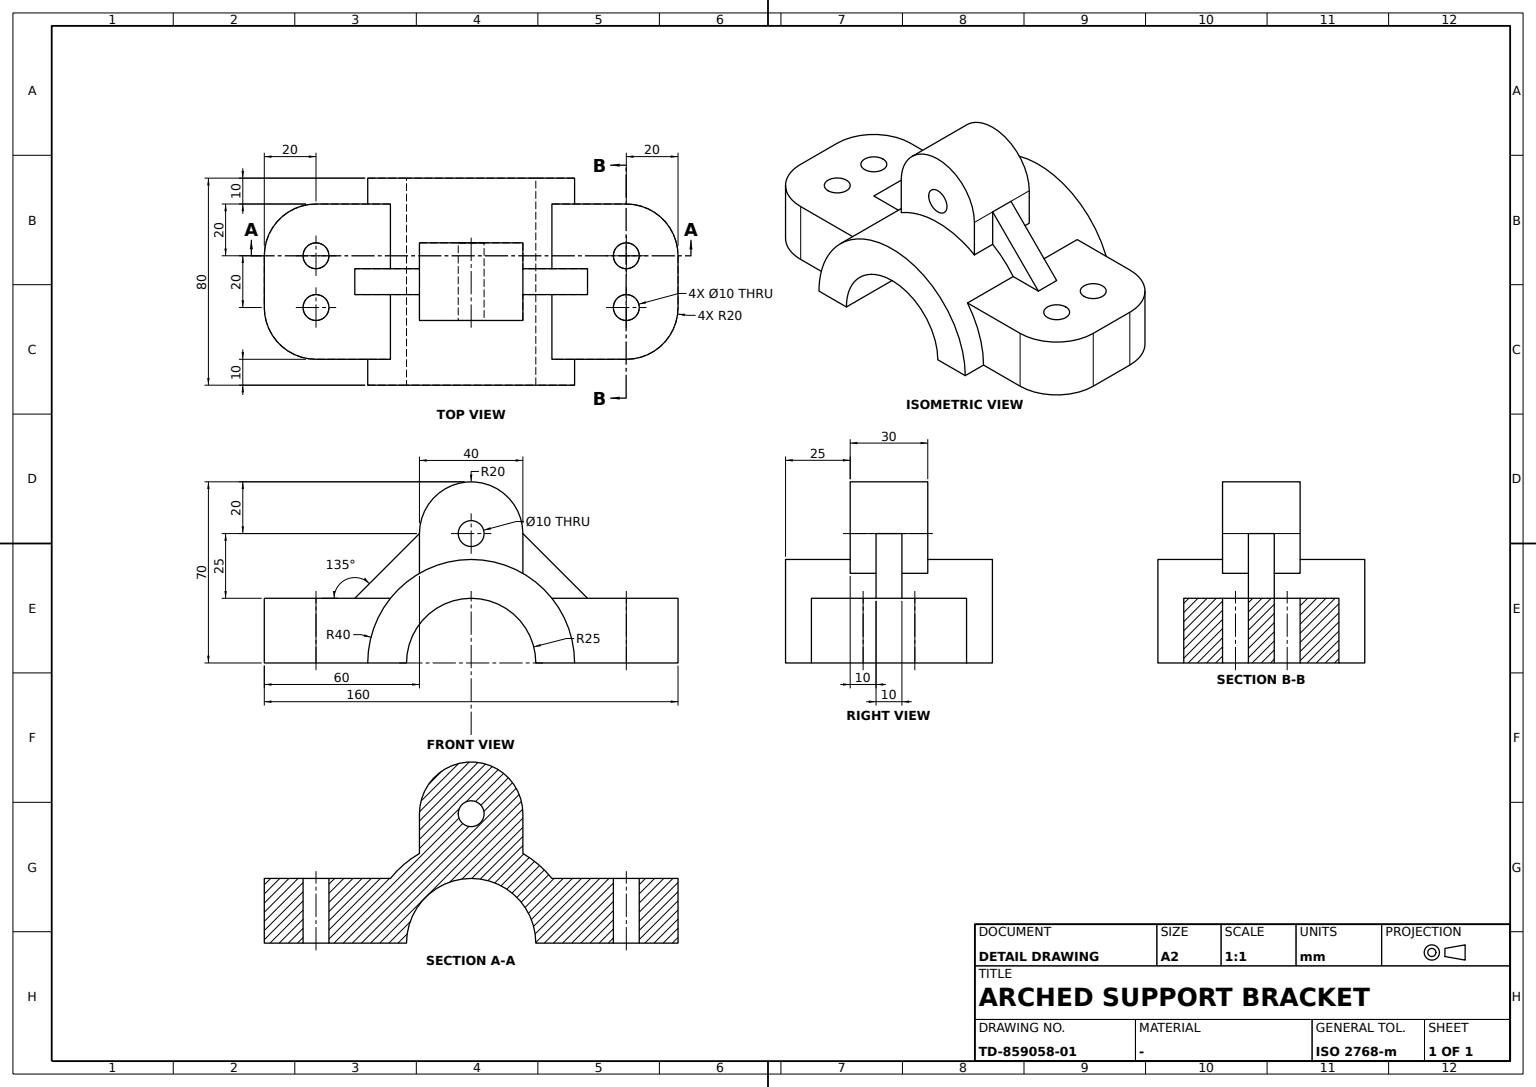
ISO-10303-21;
HEADER;
FILE_DESCRIPTION((''),'2;1');
FILE_NAME('','',(''),(''),'','','');
FILE_SCHEMA(('AUTOMOTIVE_DESIGN'));
ENDSEC;
DATA;
#1=APPLICATION_CONTEXT('');
#2=PRODUCT_CONTEXT('',#1,'mechanical');
#3=PRODUCT('','','',(#2));
#4=PRODUCT_DEFINITION_FORMATION('','',#3);
#5=PRODUCT_DEFINITION_CONTEXT('',#1,'design');
#6=PRODUCT_DEFINITION('','',#4,#5);
#7=PRODUCT_DEFINITION_SHAPE('','',#6);
#8=(LENGTH_UNIT()NAMED_UNIT(*)SI_UNIT(.MILLI.,.METRE.));
#9=(NAMED_UNIT(*)PLANE_ANGLE_UNIT()SI_UNIT($,.RADIAN.));
#10=(NAMED_UNIT(*)SI_UNIT($,.STERADIAN.)SOLID_ANGLE_UNIT());
#11=UNCERTAINTY_MEASURE_WITH_UNIT(LENGTH_MEASURE(1.E-05),#8,'distance_accuracy_value','');
#12=(GEOMETRIC_REPRESENTATION_CONTEXT(3)GLOBAL_UNCERTAINTY_ASSIGNED_CONTEXT((#11))GLOBAL_UNIT_ASSIGNED_CONTEXT((#8,#9,#10))REPRESENTATION_CONTEXT('',''));
#13=CARTESIAN_POINT('',(40.,25.,0.));
#14=VERTEX_POINT('',#13);
#15=CARTESIAN_POINT('',(40.,-25.,0.));
#16=VERTEX_POINT('',#15);
#17=CARTESIAN_POINT('',(40.,0.,0.));
#18=DIRECTION('',(1.,0.,0.));
#19=DIRECTION('',(0.,1.,0.));
#20=AXIS2_PLACEMENT_3D('',#17,#18,#19);
#21=CIRCLE('',#20,25.);
#22=EDGE_CURVE('',#14,#16,#21,.T.);
#23=ORIENTED_EDGE('',*,*,#22,.F.);
#24=CARTESIAN_POINT('',(40.,40.,0.));
#25=VERTEX_POINT('',#24);
#26=CARTESIAN_POINT('',(40.,32.5,0.));
#27=VECTOR('',#19,1000.);
#28=LINE('',#26,#27);
#29=EDGE_CURVE('',#14,#25,#28,.T.);
#30=ORIENTED_EDGE('',*,*,#29,.T.);
#31=CARTESIAN_POINT('',(40.,-40.,0.));
#32=VERTEX_POINT('',#31);
#33=CIRCLE('',#20,40.);
#34=EDGE_CURVE('',#25,#32,#33,.T.);
#35=ORIENTED_EDGE('',*,*,#34,.T.);
#36=CARTESIAN_POINT('',(40.,-32.5,0.));
#37=LINE('',#36,#27);
#38=EDGE_CURVE('',#32,#16,#37,.T.);
#39=ORIENTED_EDGE('',*,*,#38,.T.);
#40=EDGE_LOOP('',(#23,#30,#35,#39));
#41=FACE_OUTER_BOUND('',#40,.T.);
#42=PLANE('',#20);
#43=ADVANCED_FACE('',(#41),#42,.T.);
#44=CARTESIAN_POINT('',(15.,-5.,50.));
#45=VERTEX_POINT('',#44);
#46=CARTESIAN_POINT('',(-15.,-5.,50.));
#47=VERTEX_POINT('',#46);
#48=CARTESIAN_POINT('',(-13.16,-5.,50.));
#49=DIRECTION('',(-1.,0.,0.));
#50=VECTOR('',#49,1000.);
#51=LINE('',#48,#50);
#52=EDGE_CURVE('',#45,#47,#51,.T.);
#53=ORIENTED_EDGE('',*,*,#52,.F.);
#54=CARTESIAN_POINT('',(15.,5.,50.));
#55=VERTEX_POINT('',#54);
#56=CARTESIAN_POINT('',(15.,0.,50.));
#57=AXIS2_PLACEMENT_3D('',#56,#18,#19);
#58=CIRCLE('',#57,5.);
#59=EDGE_CURVE('',#45,#55,#58,.T.);
#60=ORIENTED_EDGE('',*,*,#59,.T.);
#61=CARTESIAN_POINT('',(-15.,5.,50.));
#62=VERTEX_POINT('',#61);
#63=CARTESIAN_POINT('',(-13.16,5.,50.));
#64=LINE('',#63,#50);
#65=EDGE_CURVE('',#55,#62,#64,.T.);
#66=ORIENTED_EDGE('',*,*,#65,.T.);
#67=CARTESIAN_POINT('',(-15.,0.,50.));
#68=AXIS2_PLACEMENT_3D('',#67,#18,#19);
#69=CIRCLE('',#68,5.);
#70=EDGE_CURVE('',#47,#62,#69,.T.);
#71=ORIENTED_EDGE('',*,*,#70,.F.);
#72=EDGE_LOOP('',(#53,#60,#66,#71));
#73=FACE_OUTER_BOUND('',#72,.T.);
#74=CARTESIAN_POINT('',(-13.16,0.,50.));
#75=AXIS2_PLACEMENT_3D('',#74,#49,#19);
#76=CYLINDRICAL_SURFACE('',#75,5.);
#77=ADVANCED_FACE('',(#73),#76,.F.);
#78=CARTESIAN_POINT('',(-5.,60.,0.));
#79=VERTEX_POINT('',#78);
#80=CARTESIAN_POINT('',(-15.,60.,0.));
#81=VERTEX_POINT('',#80);
#82=CARTESIAN_POINT('',(-10.,60.,0.));
#83=DIRECTION('',(0.,0.,-1.));
#84=AXIS2_PLACEMENT_3D('',#82,#83,#19);
#85=CIRCLE('',#84,5.);
#86=EDGE_CURVE('',#79,#81,#85,.T.);
#87=ORIENTED_EDGE('',*,*,#86,.T.);
#88=CARTESIAN_POINT('',(-15.,60.,25.));
#89=VERTEX_POINT('',#88);
#90=CARTESIAN_POINT('',(-15.,60.,11.84));
#91=VECTOR('',#83,1000.);
#92=LINE('',#90,#91);
#93=EDGE_CURVE('',#89,#81,#92,.T.);
#94=ORIENTED_EDGE('',*,*,#93,.F.);
#95=CARTESIAN_POINT('',(-5.,60.,25.));
#96=VERTEX_POINT('',#95);
#97=CARTESIAN_POINT('',(-10.,60.,25.));
#98=DIRECTION('',(0.,0.,1.));
#99=AXIS2_PLACEMENT_3D('',#97,#98,#18);
#100=CIRCLE('',#99,5.);
#101=EDGE_CURVE('',#89,#96,#100,.T.);
#102=ORIENTED_EDGE('',*,*,#101,.T.);
#103=CARTESIAN_POINT('',(-5.,60.,11.84));
#104=LINE('',#103,#91);
#105=EDGE_CURVE('',#96,#79,#104,.T.);
#106=ORIENTED_EDGE('',*,*,#105,.T.);
#107=EDGE_LOOP('',(#87,#94,#102,#106));
#108=FACE_OUTER_BOUND('',#107,.T.);
#109=CARTESIAN_POINT('',(-10.,60.,11.84));
#110=AXIS2_PLACEMENT_3D('',#109,#83,#18);
#111=CYLINDRICAL_SURFACE('',#110,5.);
#112=ADVANCED_FACE('',(#108),#111,.F.);
#113=CARTESIAN_POINT('',(5.,20.,50.));
#114=VERTEX_POINT('',#113);
#115=CARTESIAN_POINT('',(5.,20.,34.641016));
#116=VERTEX_POINT('',#115);
#117=CARTESIAN_POINT('',(5.,20.,42.320508));
#118=LINE('',#117,#91);
#119=EDGE_CURVE('',#114,#116,#118,.T.);
#120=ORIENTED_EDGE('',*,*,#119,.F.);
#121=CARTESIAN_POINT('',(15.,20.,50.));
#122=VERTEX_POINT('',#121);
#123=CARTESIAN_POINT('',(10.,20.,50.));
#124=VECTOR('',#18,1000.);
#125=LINE('',#123,#124);
#126=EDGE_CURVE('',#114,#122,#125,.T.);
#127=ORIENTED_EDGE('',*,*,#126,.T.);
#128=CARTESIAN_POINT('',(15.,20.,34.641016));
#129=VERTEX_POINT('',#128);
#130=CARTESIAN_POINT('',(15.,20.,42.320508));
#131=VECTOR('',#98,1000.);
#132=LINE('',#130,#131);
#133=EDGE_CURVE('',#129,#122,#132,.T.);
#134=ORIENTED_EDGE('',*,*,#133,.F.);
#135=CARTESIAN_POINT('',(0.,20.,34.641016));
#136=LINE('',#135,#124);
#137=EDGE_CURVE('',#116,#129,#136,.T.);
#138=ORIENTED_EDGE('',*,*,#137,.F.);
#139=EDGE_LOOP('',(#120,#127,#134,#138));
#140=FACE_OUTER_BOUND('',#139,.T.);
#141=CARTESIAN_POINT('',(0.,20.,50.));
#142=DIRECTION('',(0.,-1.,0.));
#143=AXIS2_PLACEMENT_3D('',#141,#142,#83);
#144=PLANE('',#143);
#145=ADVANCED_FACE('',(#140),#144,.F.);
#146=CARTESIAN_POINT('',(-30.,60.,0.));
#147=VERTEX_POINT('',#146);
#148=CARTESIAN_POINT('',(-30.,60.,25.));
#149=VERTEX_POINT('',#148);
#150=CARTESIAN_POINT('',(-30.,60.,12.5));
#151=LINE('',#150,#131);
#152=EDGE_CURVE('',#147,#149,#151,.T.);
#153=ORIENTED_EDGE('',*,*,#152,.T.);
#154=CARTESIAN_POINT('',(-10.,80.,25.));
#155=VERTEX_POINT('',#154);
#156=AXIS2_PLACEMENT_3D('',#97,#83,#142);
#157=CIRCLE('',#156,20.);
#158=EDGE_CURVE('',#149,#155,#157,.T.);
#159=ORIENTED_EDGE('',*,*,#158,.T.);
#160=CARTESIAN_POINT('',(-10.,80.,0.));
#161=VERTEX_POINT('',#160);
#162=CARTESIAN_POINT('',(-10.,80.,12.5));
#163=LINE('',#162,#131);
#164=EDGE_CURVE('',#161,#155,#163,.T.);
#165=ORIENTED_EDGE('',*,*,#164,.F.);
#166=AXIS2_PLACEMENT_3D('',#82,#98,#19);
#167=CIRCLE('',#166,20.);
#168=EDGE_CURVE('',#161,#147,#167,.T.);
#169=ORIENTED_EDGE('',*,*,#168,.T.);
#170=EDGE_LOOP('',(#153,#159,#165,#169));
#171=FACE_OUTER_BOUND('',#170,.T.);
#172=CARTESIAN_POINT('',(-10.,60.,12.5));
#173=AXIS2_PLACEMENT_3D('',#172,#83,#49);
#174=CYLINDRICAL_SURFACE('',#173,20.);
#175=ADVANCED_FACE('',(#171),#174,.T.);
#176=ORIENTED_EDGE('',*,*,#105,.F.);
#177=EDGE_CURVE('',#96,#89,#100,.T.);
#178=ORIENTED_EDGE('',*,*,#177,.T.);
#179=ORIENTED_EDGE('',*,*,#93,.T.);
#180=EDGE_CURVE('',#81,#79,#85,.T.);
#181=ORIENTED_EDGE('',*,*,#180,.T.);
#182=EDGE_LOOP('',(#176,#178,#179,#181));
#183=FACE_OUTER_BOUND('',#182,.T.);
#184=ADVANCED_FACE('',(#183),#111,.F.);
#185=ORIENTED_EDGE('',*,*,#52,.T.);
#186=EDGE_CURVE('',#62,#47,#69,.T.);
#187=ORIENTED_EDGE('',*,*,#186,.F.);
#188=ORIENTED_EDGE('',*,*,#65,.F.);
#189=EDGE_CURVE('',#55,#45,#58,.T.);
#190=ORIENTED_EDGE('',*,*,#189,.T.);
#191=EDGE_LOOP('',(#185,#187,#188,#190));
#192=FACE_OUTER_BOUND('',#191,.T.);
#193=ADVANCED_FACE('',(#192),#76,.F.);
#194=ORIENTED_EDGE('',*,*,#189,.F.);
#195=ORIENTED_EDGE('',*,*,#59,.F.);
#196=EDGE_LOOP('',(#194,#195));
#197=FACE_BOUND('',#196,.T.);
#198=CARTESIAN_POINT('',(15.,-20.,50.));
#199=VERTEX_POINT('',#198);
#200=CARTESIAN_POINT('',(15.,-20.,34.641016));
#201=VERTEX_POINT('',#200);
#202=CARTESIAN_POINT('',(15.,-20.,42.320508));
#203=LINE('',#202,#91);
#204=EDGE_CURVE('',#199,#201,#203,.T.);
#205=ORIENTED_EDGE('',*,*,#204,.T.);
#206=CARTESIAN_POINT('',(15.,0.,0.));
#207=AXIS2_PLACEMENT_3D('',#206,#49,#19);
#208=CIRCLE('',#207,40.);
#209=EDGE_CURVE('',#201,#129,#208,.T.);
#210=ORIENTED_EDGE('',*,*,#209,.T.);
#211=ORIENTED_EDGE('',*,*,#133,.T.);
#212=CIRCLE('',#57,20.);
#213=EDGE_CURVE('',#122,#199,#212,.T.);
#214=ORIENTED_EDGE('',*,*,#213,.T.);
#215=EDGE_LOOP('',(#205,#210,#211,#214));
#216=FACE_OUTER_BOUND('',#215,.T.);
#217=AXIS2_PLACEMENT_3D('',#206,#18,#19);
#218=PLANE('',#217);
#219=ADVANCED_FACE('',(#197,#216),#218,.T.);
#220=CARTESIAN_POINT('',(-15.,20.,50.));
#221=VERTEX_POINT('',#220);
#222=CARTESIAN_POINT('',(-15.,-20.,50.));
#223=VERTEX_POINT('',#222);
#224=CIRCLE('',#68,20.);
#225=EDGE_CURVE('',#221,#223,#224,.T.);
#226=ORIENTED_EDGE('',*,*,#225,.F.);
#227=CARTESIAN_POINT('',(-15.,20.,34.641016));
#228=VERTEX_POINT('',#227);
#229=CARTESIAN_POINT('',(-15.,20.,42.320508));
#230=LINE('',#229,#131);
#231=EDGE_CURVE('',#228,#221,#230,.T.);
#232=ORIENTED_EDGE('',*,*,#231,.F.);
#233=CARTESIAN_POINT('',(-15.,-20.,34.641016));
#234=VERTEX_POINT('',#233);
#235=CARTESIAN_POINT('',(-15.,0.,0.));
#236=AXIS2_PLACEMENT_3D('',#235,#49,#19);
#237=CIRCLE('',#236,40.);
#238=EDGE_CURVE('',#234,#228,#237,.T.);
#239=ORIENTED_EDGE('',*,*,#238,.F.);
#240=CARTESIAN_POINT('',(-15.,-20.,42.320508));
#241=LINE('',#240,#91);
#242=EDGE_CURVE('',#223,#234,#241,.T.);
#243=ORIENTED_EDGE('',*,*,#242,.F.);
#244=EDGE_LOOP('',(#226,#232,#239,#243));
#245=FACE_OUTER_BOUND('',#244,.T.);
#246=ORIENTED_EDGE('',*,*,#186,.T.);
#247=ORIENTED_EDGE('',*,*,#70,.T.);
#248=EDGE_LOOP('',(#246,#247));
#249=FACE_BOUND('',#248,.T.);
#250=AXIS2_PLACEMENT_3D('',#235,#18,#19);
#251=PLANE('',#250);
#252=ADVANCED_FACE('',(#245,#249),#251,.F.);
#253=CARTESIAN_POINT('',(-10.,-80.,25.));
#254=VERTEX_POINT('',#253);
#255=CARTESIAN_POINT('',(-10.,-80.,0.));
#256=VERTEX_POINT('',#255);
#257=CARTESIAN_POINT('',(-10.,-80.,12.5));
#258=LINE('',#257,#91);
#259=EDGE_CURVE('',#254,#256,#258,.T.);
#260=ORIENTED_EDGE('',*,*,#259,.T.);
#261=CARTESIAN_POINT('',(10.,-80.,0.));
#262=VERTEX_POINT('',#261);
#263=CARTESIAN_POINT('',(0.,-80.,0.));
#264=LINE('',#263,#124);
#265=EDGE_CURVE('',#256,#262,#264,.T.);
#266=ORIENTED_EDGE('',*,*,#265,.T.);
#267=CARTESIAN_POINT('',(10.,-80.,25.));
#268=VERTEX_POINT('',#267);
#269=CARTESIAN_POINT('',(10.,-80.,12.5));
#270=LINE('',#269,#91);
#271=EDGE_CURVE('',#268,#262,#270,.T.);
#272=ORIENTED_EDGE('',*,*,#271,.F.);
#273=CARTESIAN_POINT('',(0.,-80.,25.));
#274=LINE('',#273,#124);
#275=EDGE_CURVE('',#254,#268,#274,.T.);
#276=ORIENTED_EDGE('',*,*,#275,.F.);
#277=EDGE_LOOP('',(#260,#266,#272,#276));
#278=FACE_OUTER_BOUND('',#277,.T.);
#279=AXIS2_PLACEMENT_3D('',#263,#19,#98);
#280=PLANE('',#279);
#281=ADVANCED_FACE('',(#278),#280,.F.);
#282=CARTESIAN_POINT('',(-5.,-20.,50.));
#283=VERTEX_POINT('',#282);
#284=CARTESIAN_POINT('',(5.,-20.,50.));
#285=VERTEX_POINT('',#284);
#286=CARTESIAN_POINT('',(0.,-20.,50.));
#287=LINE('',#286,#124);
#288=EDGE_CURVE('',#283,#285,#287,.T.);
#289=ORIENTED_EDGE('',*,*,#288,.F.);
#290=CARTESIAN_POINT('',(-5.,-45.,25.));
#291=VERTEX_POINT('',#290);
#292=CARTESIAN_POINT('',(-5.,-32.5,37.5));
#293=DIRECTION('',(0.,-0.707106781,-0.707106781));
#294=VECTOR('',#293,1000.);
#295=LINE('',#292,#294);
#296=EDGE_CURVE('',#283,#291,#295,.T.);
#297=ORIENTED_EDGE('',*,*,#296,.T.);
#298=CARTESIAN_POINT('',(5.,-45.,25.));
#299=VERTEX_POINT('',#298);
#300=CARTESIAN_POINT('',(0.,-45.,25.));
#301=LINE('',#300,#124);
#302=EDGE_CURVE('',#291,#299,#301,.T.);
#303=ORIENTED_EDGE('',*,*,#302,.T.);
#304=CARTESIAN_POINT('',(5.,-32.5,37.5));
#305=LINE('',#304,#294);
#306=EDGE_CURVE('',#285,#299,#305,.T.);
#307=ORIENTED_EDGE('',*,*,#306,.F.);
#308=EDGE_LOOP('',(#289,#297,#303,#307));
#309=FACE_OUTER_BOUND('',#308,.T.);
#310=DIRECTION('',(0.,0.707106781,-0.707106781));
#311=DIRECTION('',(0.,0.707106781,0.707106781));
#312=AXIS2_PLACEMENT_3D('',#286,#310,#311);
#313=PLANE('',#312);
#314=ADVANCED_FACE('',(#309),#313,.F.);
#315=CARTESIAN_POINT('',(-40.,25.,0.));
#316=VERTEX_POINT('',#315);
#317=CARTESIAN_POINT('',(-40.,40.,0.));
#318=VERTEX_POINT('',#317);
#319=CARTESIAN_POINT('',(-40.,32.5,0.));
#320=LINE('',#319,#27);
#321=EDGE_CURVE('',#316,#318,#320,.T.);
#322=ORIENTED_EDGE('',*,*,#321,.F.);
#323=CARTESIAN_POINT('',(-40.,-25.,0.));
#324=VERTEX_POINT('',#323);
#325=CARTESIAN_POINT('',(-40.,0.,0.));
#326=AXIS2_PLACEMENT_3D('',#325,#18,#19);
#327=CIRCLE('',#326,25.);
#328=EDGE_CURVE('',#316,#324,#327,.T.);
#329=ORIENTED_EDGE('',*,*,#328,.T.);
#330=CARTESIAN_POINT('',(-40.,-40.,0.));
#331=VERTEX_POINT('',#330);
#332=CARTESIAN_POINT('',(-40.,-32.5,0.));
#333=LINE('',#332,#27);
#334=EDGE_CURVE('',#331,#324,#333,.T.);
#335=ORIENTED_EDGE('',*,*,#334,.F.);
#336=CIRCLE('',#326,40.);
#337=EDGE_CURVE('',#318,#331,#336,.T.);
#338=ORIENTED_EDGE('',*,*,#337,.F.);
#339=EDGE_LOOP('',(#322,#329,#335,#338));
#340=FACE_OUTER_BOUND('',#339,.T.);
#341=PLANE('',#326);
#342=ADVANCED_FACE('',(#340),#341,.F.);
#343=CARTESIAN_POINT('',(-30.,-60.,25.));
#344=VERTEX_POINT('',#343);
#345=CARTESIAN_POINT('',(-30.,-60.,0.));
#346=VERTEX_POINT('',#345);
#347=CARTESIAN_POINT('',(-30.,-60.,12.5));
#348=LINE('',#347,#91);
#349=EDGE_CURVE('',#344,#346,#348,.T.);
#350=ORIENTED_EDGE('',*,*,#349,.F.);
#351=CARTESIAN_POINT('',(-30.,-31.22499,25.));
#352=VERTEX_POINT('',#351);
#353=CARTESIAN_POINT('',(-30.,-45.612495,25.));
#354=VECTOR('',#142,1000.);
#355=LINE('',#353,#354);
#356=EDGE_CURVE('',#352,#344,#355,.T.);
#357=ORIENTED_EDGE('',*,*,#356,.F.);
#358=CARTESIAN_POINT('',(-30.,-40.,0.));
#359=VERTEX_POINT('',#358);
#360=CARTESIAN_POINT('',(-30.,0.,0.));
#361=AXIS2_PLACEMENT_3D('',#360,#18,#19);
#362=CIRCLE('',#361,40.);
#363=EDGE_CURVE('',#352,#359,#362,.T.);
#364=ORIENTED_EDGE('',*,*,#363,.T.);
#365=CARTESIAN_POINT('',(-30.,-50.,0.));
#366=LINE('',#365,#27);
#367=EDGE_CURVE('',#346,#359,#366,.T.);
#368=ORIENTED_EDGE('',*,*,#367,.F.);
#369=EDGE_LOOP('',(#350,#357,#364,#368));
#370=FACE_OUTER_BOUND('',#369,.T.);
#371=PLANE('',#361);
#372=ADVANCED_FACE('',(#370),#371,.F.);
#373=CARTESIAN_POINT('',(5.,60.,25.));
#374=VERTEX_POINT('',#373);
#375=CARTESIAN_POINT('',(15.,60.,25.));
#376=VERTEX_POINT('',#375);
#377=CARTESIAN_POINT('',(10.,60.,25.));
#378=AXIS2_PLACEMENT_3D('',#377,#98,#18);
#379=CIRCLE('',#378,5.);
#380=EDGE_CURVE('',#374,#376,#379,.T.);
#381=ORIENTED_EDGE('',*,*,#380,.T.);
#382=CARTESIAN_POINT('',(15.,60.,0.));
#383=VERTEX_POINT('',#382);
#384=CARTESIAN_POINT('',(15.,60.,11.84));
#385=LINE('',#384,#91);
#386=EDGE_CURVE('',#376,#383,#385,.T.);
#387=ORIENTED_EDGE('',*,*,#386,.T.);
#388=CARTESIAN_POINT('',(5.,60.,0.));
#389=VERTEX_POINT('',#388);
#390=CARTESIAN_POINT('',(10.,60.,0.));
#391=AXIS2_PLACEMENT_3D('',#390,#83,#19);
#392=CIRCLE('',#391,5.);
#393=EDGE_CURVE('',#383,#389,#392,.T.);
#394=ORIENTED_EDGE('',*,*,#393,.T.);
#395=CARTESIAN_POINT('',(5.,60.,11.84));
#396=LINE('',#395,#91);
#397=EDGE_CURVE('',#374,#389,#396,.T.);
#398=ORIENTED_EDGE('',*,*,#397,.F.);
#399=EDGE_LOOP('',(#381,#387,#394,#398));
#400=FACE_OUTER_BOUND('',#399,.T.);
#401=CARTESIAN_POINT('',(10.,60.,11.84));
#402=AXIS2_PLACEMENT_3D('',#401,#83,#18);
#403=CYLINDRICAL_SURFACE('',#402,5.);
#404=ADVANCED_FACE('',(#400),#403,.F.);
#405=CARTESIAN_POINT('',(-5.,45.,25.));
#406=VERTEX_POINT('',#405);
#407=CARTESIAN_POINT('',(-5.,31.22499,25.));
#408=VERTEX_POINT('',#407);
#409=CARTESIAN_POINT('',(-5.,38.112495,25.));
#410=LINE('',#409,#354);
#411=EDGE_CURVE('',#406,#408,#410,.T.);
#412=ORIENTED_EDGE('',*,*,#411,.T.);
#413=CARTESIAN_POINT('',(-5.,20.,34.641016));
#414=VERTEX_POINT('',#413);
#415=CARTESIAN_POINT('',(-5.,0.,0.));
#416=AXIS2_PLACEMENT_3D('',#415,#18,#19);
#417=CIRCLE('',#416,40.);
#418=EDGE_CURVE('',#408,#414,#417,.T.);
#419=ORIENTED_EDGE('',*,*,#418,.T.);
#420=CARTESIAN_POINT('',(-5.,20.,50.));
#421=VERTEX_POINT('',#420);
#422=CARTESIAN_POINT('',(-5.,20.,42.320508));
#423=LINE('',#422,#91);
#424=EDGE_CURVE('',#421,#414,#423,.T.);
#425=ORIENTED_EDGE('',*,*,#424,.F.);
#426=CARTESIAN_POINT('',(-5.,32.5,37.5));
#427=VECTOR('',#310,1000.);
#428=LINE('',#426,#427);
#429=EDGE_CURVE('',#421,#406,#428,.T.);
#430=ORIENTED_EDGE('',*,*,#429,.T.);
#431=EDGE_LOOP('',(#412,#419,#425,#430));
#432=FACE_OUTER_BOUND('',#431,.T.);
#433=PLANE('',#416);
#434=ADVANCED_FACE('',(#432),#433,.F.);
#435=CARTESIAN_POINT('',(5.,-20.,34.641016));
#436=VERTEX_POINT('',#435);
#437=CARTESIAN_POINT('',(5.,-31.22499,25.));
#438=VERTEX_POINT('',#437);
#439=CARTESIAN_POINT('',(5.,0.,0.));
#440=AXIS2_PLACEMENT_3D('',#439,#18,#19);
#441=CIRCLE('',#440,40.);
#442=EDGE_CURVE('',#436,#438,#441,.T.);
#443=ORIENTED_EDGE('',*,*,#442,.F.);
#444=CARTESIAN_POINT('',(5.,-20.,42.320508));
#445=LINE('',#444,#91);
#446=EDGE_CURVE('',#285,#436,#445,.T.);
#447=ORIENTED_EDGE('',*,*,#446,.F.);
#448=ORIENTED_EDGE('',*,*,#306,.T.);
#449=CARTESIAN_POINT('',(5.,-38.112495,25.));
#450=LINE('',#449,#354);
#451=EDGE_CURVE('',#438,#299,#450,.T.);
#452=ORIENTED_EDGE('',*,*,#451,.F.);
#453=EDGE_LOOP('',(#443,#447,#448,#452));
#454=FACE_OUTER_BOUND('',#453,.T.);
#455=PLANE('',#440);
#456=ADVANCED_FACE('',(#454),#455,.T.);
#457=ORIENTED_EDGE('',*,*,#386,.F.);
#458=EDGE_CURVE('',#376,#374,#379,.T.);
#459=ORIENTED_EDGE('',*,*,#458,.T.);
#460=ORIENTED_EDGE('',*,*,#397,.T.);
#461=EDGE_CURVE('',#389,#383,#392,.T.);
#462=ORIENTED_EDGE('',*,*,#461,.T.);
#463=EDGE_LOOP('',(#457,#459,#460,#462));
#464=FACE_OUTER_BOUND('',#463,.T.);
#465=ADVANCED_FACE('',(#464),#403,.F.);
#466=CARTESIAN_POINT('',(5.,45.,25.));
#467=VERTEX_POINT('',#466);
#468=CARTESIAN_POINT('',(5.,32.5,37.5));
#469=LINE('',#468,#427);
#470=EDGE_CURVE('',#114,#467,#469,.T.);
#471=ORIENTED_EDGE('',*,*,#470,.F.);
#472=ORIENTED_EDGE('',*,*,#119,.T.);
#473=CARTESIAN_POINT('',(5.,31.22499,25.));
#474=VERTEX_POINT('',#473);
#475=EDGE_CURVE('',#474,#116,#441,.T.);
#476=ORIENTED_EDGE('',*,*,#475,.F.);
#477=CARTESIAN_POINT('',(5.,38.112495,25.));
#478=LINE('',#477,#354);
#479=EDGE_CURVE('',#467,#474,#478,.T.);
#480=ORIENTED_EDGE('',*,*,#479,.F.);
#481=EDGE_LOOP('',(#471,#472,#476,#480));
#482=FACE_OUTER_BOUND('',#481,.T.);
#483=ADVANCED_FACE('',(#482),#455,.T.);
#484=CARTESIAN_POINT('',(0.,-25.,0.));
#485=LINE('',#484,#50);
#486=EDGE_CURVE('',#16,#324,#485,.T.);
#487=ORIENTED_EDGE('',*,*,#486,.T.);
#488=ORIENTED_EDGE('',*,*,#328,.F.);
#489=CARTESIAN_POINT('',(-0.66,25.,0.));
#490=LINE('',#489,#50);
#491=EDGE_CURVE('',#14,#316,#490,.T.);
#492=ORIENTED_EDGE('',*,*,#491,.F.);
#493=ORIENTED_EDGE('',*,*,#22,.T.);
#494=EDGE_LOOP('',(#487,#488,#492,#493));
#495=FACE_OUTER_BOUND('',#494,.T.);
#496=CARTESIAN_POINT('',(-0.66,0.,0.));
#497=AXIS2_PLACEMENT_3D('',#496,#49,#19);
#498=CYLINDRICAL_SURFACE('',#497,25.);
#499=ADVANCED_FACE('',(#495),#498,.F.);
#500=CARTESIAN_POINT('',(30.,-60.,25.));
#501=VERTEX_POINT('',#500);
#502=CARTESIAN_POINT('',(30.,-60.,0.));
#503=VERTEX_POINT('',#502);
#504=CARTESIAN_POINT('',(30.,-60.,12.5));
#505=LINE('',#504,#91);
#506=EDGE_CURVE('',#501,#503,#505,.T.);
#507=ORIENTED_EDGE('',*,*,#506,.F.);
#508=CARTESIAN_POINT('',(10.,-60.,25.));
#509=AXIS2_PLACEMENT_3D('',#508,#83,#142);
#510=CIRCLE('',#509,20.);
#511=EDGE_CURVE('',#501,#268,#510,.T.);
#512=ORIENTED_EDGE('',*,*,#511,.T.);
#513=ORIENTED_EDGE('',*,*,#271,.T.);
#514=CARTESIAN_POINT('',(10.,-60.,0.));
#515=AXIS2_PLACEMENT_3D('',#514,#98,#19);
#516=CIRCLE('',#515,20.);
#517=EDGE_CURVE('',#262,#503,#516,.T.);
#518=ORIENTED_EDGE('',*,*,#517,.T.);
#519=EDGE_LOOP('',(#507,#512,#513,#518));
#520=FACE_OUTER_BOUND('',#519,.T.);
#521=CARTESIAN_POINT('',(10.,-60.,12.5));
#522=AXIS2_PLACEMENT_3D('',#521,#83,#142);
#523=CYLINDRICAL_SURFACE('',#522,20.);
#524=ADVANCED_FACE('',(#520),#523,.T.);
#525=CARTESIAN_POINT('',(30.,31.22499,25.));
#526=VERTEX_POINT('',#525);
#527=CARTESIAN_POINT('',(17.5,31.22499,25.));
#528=LINE('',#527,#124);
#529=EDGE_CURVE('',#474,#526,#528,.T.);
#530=ORIENTED_EDGE('',*,*,#529,.T.);
#531=CARTESIAN_POINT('',(30.,60.,25.));
#532=VERTEX_POINT('',#531);
#533=CARTESIAN_POINT('',(30.,45.612495,25.));
#534=LINE('',#533,#354);
#535=EDGE_CURVE('',#532,#526,#534,.T.);
#536=ORIENTED_EDGE('',*,*,#535,.F.);
#537=CARTESIAN_POINT('',(10.,80.,25.));
#538=VERTEX_POINT('',#537);
#539=AXIS2_PLACEMENT_3D('',#377,#83,#142);
#540=CIRCLE('',#539,20.);
#541=EDGE_CURVE('',#538,#532,#540,.T.);
#542=ORIENTED_EDGE('',*,*,#541,.F.);
#543=CARTESIAN_POINT('',(0.,80.,25.));
#544=LINE('',#543,#124);
#545=EDGE_CURVE('',#155,#538,#544,.T.);
#546=ORIENTED_EDGE('',*,*,#545,.F.);
#547=ORIENTED_EDGE('',*,*,#158,.F.);
#548=CARTESIAN_POINT('',(-30.,31.22499,25.));
#549=VERTEX_POINT('',#548);
#550=CARTESIAN_POINT('',(-30.,45.612495,25.));
#551=LINE('',#550,#354);
#552=EDGE_CURVE('',#149,#549,#551,.T.);
#553=ORIENTED_EDGE('',*,*,#552,.T.);
#554=CARTESIAN_POINT('',(-17.5,31.22499,25.));
#555=LINE('',#554,#124);
#556=EDGE_CURVE('',#549,#408,#555,.T.);
#557=ORIENTED_EDGE('',*,*,#556,.T.);
#558=ORIENTED_EDGE('',*,*,#411,.F.);
#559=CARTESIAN_POINT('',(0.,45.,25.));
#560=LINE('',#559,#124);
#561=EDGE_CURVE('',#406,#467,#560,.T.);
#562=ORIENTED_EDGE('',*,*,#561,.T.);
#563=ORIENTED_EDGE('',*,*,#479,.T.);
#564=EDGE_LOOP('',(#530,#536,#542,#546,#547,#553,#557,#558,#562,#563));
#565=FACE_OUTER_BOUND('',#564,.T.);
#566=ORIENTED_EDGE('',*,*,#380,.F.);
#567=ORIENTED_EDGE('',*,*,#458,.F.);
#568=EDGE_LOOP('',(#566,#567));
#569=FACE_BOUND('',#568,.T.);
#570=ORIENTED_EDGE('',*,*,#101,.F.);
#571=ORIENTED_EDGE('',*,*,#177,.F.);
#572=EDGE_LOOP('',(#570,#571));
#573=FACE_BOUND('',#572,.T.);
#574=AXIS2_PLACEMENT_3D('',#543,#98,#142);
#575=PLANE('',#574);
#576=ADVANCED_FACE('',(#565,#569,#573),#575,.T.);
#577=ORIENTED_EDGE('',*,*,#296,.F.);
#578=CARTESIAN_POINT('',(-5.,-20.,34.641016));
#579=VERTEX_POINT('',#578);
#580=CARTESIAN_POINT('',(-5.,-20.,42.320508));
#581=LINE('',#580,#91);
#582=EDGE_CURVE('',#283,#579,#581,.T.);
#583=ORIENTED_EDGE('',*,*,#582,.T.);
#584=CARTESIAN_POINT('',(-5.,-31.22499,25.));
#585=VERTEX_POINT('',#584);
#586=EDGE_CURVE('',#579,#585,#417,.T.);
#587=ORIENTED_EDGE('',*,*,#586,.T.);
#588=CARTESIAN_POINT('',(-5.,-38.112495,25.));
#589=LINE('',#588,#354);
#590=EDGE_CURVE('',#585,#291,#589,.T.);
#591=ORIENTED_EDGE('',*,*,#590,.T.);
#592=EDGE_LOOP('',(#577,#583,#587,#591));
#593=FACE_OUTER_BOUND('',#592,.T.);
#594=ADVANCED_FACE('',(#593),#433,.F.);
#595=ORIENTED_EDGE('',*,*,#561,.F.);
#596=ORIENTED_EDGE('',*,*,#429,.F.);
#597=LINE('',#141,#124);
#598=EDGE_CURVE('',#421,#114,#597,.T.);
#599=ORIENTED_EDGE('',*,*,#598,.T.);
#600=ORIENTED_EDGE('',*,*,#470,.T.);
#601=EDGE_LOOP('',(#595,#596,#599,#600));
#602=FACE_OUTER_BOUND('',#601,.T.);
#603=DIRECTION('',(0.,-0.707106781,0.707106781));
#604=AXIS2_PLACEMENT_3D('',#141,#311,#603);
#605=PLANE('',#604);
#606=ADVANCED_FACE('',(#602),#605,.T.);
#607=CARTESIAN_POINT('',(10.,80.,0.));
#608=VERTEX_POINT('',#607);
#609=CARTESIAN_POINT('',(0.,80.,0.));
#610=LINE('',#609,#124);
#611=EDGE_CURVE('',#161,#608,#610,.T.);
#612=ORIENTED_EDGE('',*,*,#611,.F.);
#613=ORIENTED_EDGE('',*,*,#164,.T.);
#614=ORIENTED_EDGE('',*,*,#545,.T.);
#615=CARTESIAN_POINT('',(10.,80.,12.5));
#616=LINE('',#615,#131);
#617=EDGE_CURVE('',#608,#538,#616,.T.);
#618=ORIENTED_EDGE('',*,*,#617,.F.);
#619=EDGE_LOOP('',(#612,#613,#614,#618));
#620=FACE_OUTER_BOUND('',#619,.T.);
#621=AXIS2_PLACEMENT_3D('',#609,#19,#98);
#622=PLANE('',#621);
#623=ADVANCED_FACE('',(#620),#622,.T.);
#624=ORIENTED_EDGE('',*,*,#541,.T.);
#625=CARTESIAN_POINT('',(30.,60.,0.));
#626=VERTEX_POINT('',#625);
#627=CARTESIAN_POINT('',(30.,60.,12.5));
#628=LINE('',#627,#131);
#629=EDGE_CURVE('',#626,#532,#628,.T.);
#630=ORIENTED_EDGE('',*,*,#629,.F.);
#631=AXIS2_PLACEMENT_3D('',#390,#98,#19);
#632=CIRCLE('',#631,20.);
#633=EDGE_CURVE('',#626,#608,#632,.T.);
#634=ORIENTED_EDGE('',*,*,#633,.T.);
#635=ORIENTED_EDGE('',*,*,#617,.T.);
#636=EDGE_LOOP('',(#624,#630,#634,#635));
#637=FACE_OUTER_BOUND('',#636,.T.);
#638=CARTESIAN_POINT('',(10.,60.,12.5));
#639=AXIS2_PLACEMENT_3D('',#638,#83,#19);
#640=CYLINDRICAL_SURFACE('',#639,20.);
#641=ADVANCED_FACE('',(#637),#640,.T.);
#642=CARTESIAN_POINT('',(5.,-60.,25.));
#643=VERTEX_POINT('',#642);
#644=CARTESIAN_POINT('',(15.,-60.,25.));
#645=VERTEX_POINT('',#644);
#646=AXIS2_PLACEMENT_3D('',#508,#98,#18);
#647=CIRCLE('',#646,5.);
#648=EDGE_CURVE('',#643,#645,#647,.T.);
#649=ORIENTED_EDGE('',*,*,#648,.T.);
#650=CARTESIAN_POINT('',(15.,-60.,0.));
#651=VERTEX_POINT('',#650);
#652=CARTESIAN_POINT('',(15.,-60.,11.84));
#653=LINE('',#652,#91);
#654=EDGE_CURVE('',#645,#651,#653,.T.);
#655=ORIENTED_EDGE('',*,*,#654,.T.);
#656=CARTESIAN_POINT('',(5.,-60.,0.));
#657=VERTEX_POINT('',#656);
#658=AXIS2_PLACEMENT_3D('',#514,#83,#19);
#659=CIRCLE('',#658,5.);
#660=EDGE_CURVE('',#651,#657,#659,.T.);
#661=ORIENTED_EDGE('',*,*,#660,.T.);
#662=CARTESIAN_POINT('',(5.,-60.,11.84));
#663=LINE('',#662,#91);
#664=EDGE_CURVE('',#643,#657,#663,.T.);
#665=ORIENTED_EDGE('',*,*,#664,.F.);
#666=EDGE_LOOP('',(#649,#655,#661,#665));
#667=FACE_OUTER_BOUND('',#666,.T.);
#668=CARTESIAN_POINT('',(10.,-60.,11.84));
#669=AXIS2_PLACEMENT_3D('',#668,#83,#18);
#670=CYLINDRICAL_SURFACE('',#669,5.);
#671=ADVANCED_FACE('',(#667),#670,.F.);
#672=EDGE_CURVE('',#657,#651,#659,.T.);
#673=ORIENTED_EDGE('',*,*,#672,.T.);
#674=ORIENTED_EDGE('',*,*,#654,.F.);
#675=EDGE_CURVE('',#645,#643,#647,.T.);
#676=ORIENTED_EDGE('',*,*,#675,.T.);
#677=ORIENTED_EDGE('',*,*,#664,.T.);
#678=EDGE_LOOP('',(#673,#674,#676,#677));
#679=FACE_OUTER_BOUND('',#678,.T.);
#680=ADVANCED_FACE('',(#679),#670,.F.);
#681=CARTESIAN_POINT('',(30.,-40.,0.));
#682=VERTEX_POINT('',#681);
#683=CARTESIAN_POINT('',(35.,-40.,0.));
#684=LINE('',#683,#124);
#685=EDGE_CURVE('',#682,#32,#684,.T.);
#686=ORIENTED_EDGE('',*,*,#685,.T.);
#687=ORIENTED_EDGE('',*,*,#34,.F.);
#688=CARTESIAN_POINT('',(30.,40.,0.));
#689=VERTEX_POINT('',#688);
#690=CARTESIAN_POINT('',(35.,40.,0.));
#691=LINE('',#690,#124);
#692=EDGE_CURVE('',#689,#25,#691,.T.);
#693=ORIENTED_EDGE('',*,*,#692,.F.);
#694=CARTESIAN_POINT('',(30.,0.,0.));
#695=AXIS2_PLACEMENT_3D('',#694,#18,#19);
#696=CIRCLE('',#695,40.);
#697=EDGE_CURVE('',#689,#526,#696,.T.);
#698=ORIENTED_EDGE('',*,*,#697,.T.);
#699=ORIENTED_EDGE('',*,*,#529,.F.);
#700=ORIENTED_EDGE('',*,*,#475,.T.);
#701=ORIENTED_EDGE('',*,*,#137,.T.);
#702=ORIENTED_EDGE('',*,*,#209,.F.);
#703=CARTESIAN_POINT('',(10.,-20.,34.641016));
#704=LINE('',#703,#124);
#705=EDGE_CURVE('',#436,#201,#704,.T.);
#706=ORIENTED_EDGE('',*,*,#705,.F.);
#707=ORIENTED_EDGE('',*,*,#442,.T.);
#708=CARTESIAN_POINT('',(30.,-31.22499,25.));
#709=VERTEX_POINT('',#708);
#710=CARTESIAN_POINT('',(17.5,-31.22499,25.));
#711=LINE('',#710,#124);
#712=EDGE_CURVE('',#438,#709,#711,.T.);
#713=ORIENTED_EDGE('',*,*,#712,.T.);
#714=EDGE_CURVE('',#709,#682,#696,.T.);
#715=ORIENTED_EDGE('',*,*,#714,.T.);
#716=EDGE_LOOP('',(#686,#687,#693,#698,#699,#700,#701,#702,#706,#707,#713,#715));
#717=FACE_OUTER_BOUND('',#716,.T.);
#718=CARTESIAN_POINT('',(0.,0.,0.));
#719=AXIS2_PLACEMENT_3D('',#718,#49,#19);
#720=CYLINDRICAL_SURFACE('',#719,40.);
#721=ADVANCED_FACE('',(#717),#720,.T.);
#722=CARTESIAN_POINT('',(-15.,-60.,0.));
#723=VERTEX_POINT('',#722);
#724=CARTESIAN_POINT('',(-5.,-60.,0.));
#725=VERTEX_POINT('',#724);
#726=CARTESIAN_POINT('',(-10.,-60.,0.));
#727=AXIS2_PLACEMENT_3D('',#726,#83,#19);
#728=CIRCLE('',#727,5.);
#729=EDGE_CURVE('',#723,#725,#728,.T.);
#730=ORIENTED_EDGE('',*,*,#729,.T.);
#731=CARTESIAN_POINT('',(-5.,-60.,25.));
#732=VERTEX_POINT('',#731);
#733=CARTESIAN_POINT('',(-5.,-60.,11.84));
#734=LINE('',#733,#91);
#735=EDGE_CURVE('',#732,#725,#734,.T.);
#736=ORIENTED_EDGE('',*,*,#735,.F.);
#737=CARTESIAN_POINT('',(-15.,-60.,25.));
#738=VERTEX_POINT('',#737);
#739=CARTESIAN_POINT('',(-10.,-60.,25.));
#740=AXIS2_PLACEMENT_3D('',#739,#98,#18);
#741=CIRCLE('',#740,5.);
#742=EDGE_CURVE('',#732,#738,#741,.T.);
#743=ORIENTED_EDGE('',*,*,#742,.T.);
#744=CARTESIAN_POINT('',(-15.,-60.,11.84));
#745=LINE('',#744,#91);
#746=EDGE_CURVE('',#738,#723,#745,.T.);
#747=ORIENTED_EDGE('',*,*,#746,.T.);
#748=EDGE_LOOP('',(#730,#736,#743,#747));
#749=FACE_OUTER_BOUND('',#748,.T.);
#750=CARTESIAN_POINT('',(-10.,-60.,11.84));
#751=AXIS2_PLACEMENT_3D('',#750,#83,#18);
#752=CYLINDRICAL_SURFACE('',#751,5.);
#753=ADVANCED_FACE('',(#749),#752,.F.);
#754=CARTESIAN_POINT('',(-30.,40.,0.));
#755=VERTEX_POINT('',#754);
#756=CARTESIAN_POINT('',(-35.,40.,0.));
#757=LINE('',#756,#124);
#758=EDGE_CURVE('',#318,#755,#757,.T.);
#759=ORIENTED_EDGE('',*,*,#758,.F.);
#760=ORIENTED_EDGE('',*,*,#337,.T.);
#761=CARTESIAN_POINT('',(-35.,-40.,0.));
#762=LINE('',#761,#124);
#763=EDGE_CURVE('',#331,#359,#762,.T.);
#764=ORIENTED_EDGE('',*,*,#763,.T.);
#765=ORIENTED_EDGE('',*,*,#363,.F.);
#766=CARTESIAN_POINT('',(-17.5,-31.22499,25.));
#767=LINE('',#766,#124);
#768=EDGE_CURVE('',#352,#585,#767,.T.);
#769=ORIENTED_EDGE('',*,*,#768,.T.);
#770=ORIENTED_EDGE('',*,*,#586,.F.);
#771=CARTESIAN_POINT('',(-10.,-20.,34.641016));
#772=LINE('',#771,#124);
#773=EDGE_CURVE('',#234,#579,#772,.T.);
#774=ORIENTED_EDGE('',*,*,#773,.F.);
#775=ORIENTED_EDGE('',*,*,#238,.T.);
#776=EDGE_CURVE('',#228,#414,#136,.T.);
#777=ORIENTED_EDGE('',*,*,#776,.T.);
#778=ORIENTED_EDGE('',*,*,#418,.F.);
#779=ORIENTED_EDGE('',*,*,#556,.F.);
#780=EDGE_CURVE('',#755,#549,#362,.T.);
#781=ORIENTED_EDGE('',*,*,#780,.F.);
#782=EDGE_LOOP('',(#759,#760,#764,#765,#769,#770,#774,#775,#777,#778,#779,#781));
#783=FACE_OUTER_BOUND('',#782,.T.);
#784=ADVANCED_FACE('',(#783),#720,.T.);
#785=CARTESIAN_POINT('',(10.,-20.,50.));
#786=LINE('',#785,#124);
#787=EDGE_CURVE('',#285,#199,#786,.T.);
#788=ORIENTED_EDGE('',*,*,#787,.F.);
#789=ORIENTED_EDGE('',*,*,#446,.T.);
#790=ORIENTED_EDGE('',*,*,#705,.T.);
#791=ORIENTED_EDGE('',*,*,#204,.F.);
#792=EDGE_LOOP('',(#788,#789,#790,#791));
#793=FACE_OUTER_BOUND('',#792,.T.);
#794=AXIS2_PLACEMENT_3D('',#286,#142,#83);
#795=PLANE('',#794);
#796=ADVANCED_FACE('',(#793),#795,.T.);
#797=ORIENTED_EDGE('',*,*,#535,.T.);
#798=ORIENTED_EDGE('',*,*,#697,.F.);
#799=CARTESIAN_POINT('',(30.,50.,0.));
#800=LINE('',#799,#27);
#801=EDGE_CURVE('',#689,#626,#800,.T.);
#802=ORIENTED_EDGE('',*,*,#801,.T.);
#803=ORIENTED_EDGE('',*,*,#629,.T.);
#804=EDGE_LOOP('',(#797,#798,#802,#803));
#805=FACE_OUTER_BOUND('',#804,.T.);
#806=PLANE('',#695);
#807=ADVANCED_FACE('',(#805),#806,.T.);
#808=CARTESIAN_POINT('',(-10.,-20.,50.));
#809=LINE('',#808,#124);
#810=EDGE_CURVE('',#223,#283,#809,.T.);
#811=ORIENTED_EDGE('',*,*,#810,.F.);
#812=ORIENTED_EDGE('',*,*,#242,.T.);
#813=ORIENTED_EDGE('',*,*,#773,.T.);
#814=ORIENTED_EDGE('',*,*,#582,.F.);
#815=EDGE_LOOP('',(#811,#812,#813,#814));
#816=FACE_OUTER_BOUND('',#815,.T.);
#817=ADVANCED_FACE('',(#816),#795,.T.);
#818=ORIENTED_EDGE('',*,*,#672,.F.);
#819=ORIENTED_EDGE('',*,*,#660,.F.);
#820=EDGE_LOOP('',(#818,#819));
#821=FACE_BOUND('',#820,.T.);
#822=ORIENTED_EDGE('',*,*,#729,.F.);
#823=EDGE_CURVE('',#725,#723,#728,.T.);
#824=ORIENTED_EDGE('',*,*,#823,.F.);
#825=EDGE_LOOP('',(#822,#824));
#826=FACE_BOUND('',#825,.T.);
#827=ORIENTED_EDGE('',*,*,#265,.F.);
#828=AXIS2_PLACEMENT_3D('',#726,#98,#19);
#829=CIRCLE('',#828,20.);
#830=EDGE_CURVE('',#346,#256,#829,.T.);
#831=ORIENTED_EDGE('',*,*,#830,.F.);
#832=ORIENTED_EDGE('',*,*,#367,.T.);
#833=ORIENTED_EDGE('',*,*,#763,.F.);
#834=ORIENTED_EDGE('',*,*,#334,.T.);
#835=ORIENTED_EDGE('',*,*,#486,.F.);
#836=ORIENTED_EDGE('',*,*,#38,.F.);
#837=ORIENTED_EDGE('',*,*,#685,.F.);
#838=CARTESIAN_POINT('',(30.,-50.,0.));
#839=LINE('',#838,#27);
#840=EDGE_CURVE('',#503,#682,#839,.T.);
#841=ORIENTED_EDGE('',*,*,#840,.F.);
#842=ORIENTED_EDGE('',*,*,#517,.F.);
#843=EDGE_LOOP('',(#827,#831,#832,#833,#834,#835,#836,#837,#841,#842));
#844=FACE_OUTER_BOUND('',#843,.T.);
#845=AXIS2_PLACEMENT_3D('',#263,#83,#19);
#846=PLANE('',#845);
#847=ADVANCED_FACE('',(#821,#826,#844),#846,.T.);
#848=CARTESIAN_POINT('',(-30.,50.,0.));
#849=LINE('',#848,#27);
#850=EDGE_CURVE('',#755,#147,#849,.T.);
#851=ORIENTED_EDGE('',*,*,#850,.F.);
#852=ORIENTED_EDGE('',*,*,#780,.T.);
#853=ORIENTED_EDGE('',*,*,#552,.F.);
#854=ORIENTED_EDGE('',*,*,#152,.F.);
#855=EDGE_LOOP('',(#851,#852,#853,#854));
#856=FACE_OUTER_BOUND('',#855,.T.);
#857=ADVANCED_FACE('',(#856),#371,.F.);
#858=ORIENTED_EDGE('',*,*,#742,.F.);
#859=EDGE_CURVE('',#738,#732,#741,.T.);
#860=ORIENTED_EDGE('',*,*,#859,.F.);
#861=EDGE_LOOP('',(#858,#860));
#862=FACE_BOUND('',#861,.T.);
#863=ORIENTED_EDGE('',*,*,#675,.F.);
#864=ORIENTED_EDGE('',*,*,#648,.F.);
#865=EDGE_LOOP('',(#863,#864));
#866=FACE_BOUND('',#865,.T.);
#867=ORIENTED_EDGE('',*,*,#302,.F.);
#868=ORIENTED_EDGE('',*,*,#590,.F.);
#869=ORIENTED_EDGE('',*,*,#768,.F.);
#870=ORIENTED_EDGE('',*,*,#356,.T.);
#871=AXIS2_PLACEMENT_3D('',#739,#83,#142);
#872=CIRCLE('',#871,20.);
#873=EDGE_CURVE('',#254,#344,#872,.T.);
#874=ORIENTED_EDGE('',*,*,#873,.F.);
#875=ORIENTED_EDGE('',*,*,#275,.T.);
#876=ORIENTED_EDGE('',*,*,#511,.F.);
#877=CARTESIAN_POINT('',(30.,-45.612495,25.));
#878=LINE('',#877,#354);
#879=EDGE_CURVE('',#709,#501,#878,.T.);
#880=ORIENTED_EDGE('',*,*,#879,.F.);
#881=ORIENTED_EDGE('',*,*,#712,.F.);
#882=ORIENTED_EDGE('',*,*,#451,.T.);
#883=EDGE_LOOP('',(#867,#868,#869,#870,#874,#875,#876,#880,#881,#882));
#884=FACE_OUTER_BOUND('',#883,.T.);
#885=ADVANCED_FACE('',(#862,#866,#884),#575,.T.);
#886=ORIENTED_EDGE('',*,*,#231,.T.);
#887=CARTESIAN_POINT('',(-10.,20.,50.));
#888=LINE('',#887,#124);
#889=EDGE_CURVE('',#221,#421,#888,.T.);
#890=ORIENTED_EDGE('',*,*,#889,.T.);
#891=ORIENTED_EDGE('',*,*,#424,.T.);
#892=ORIENTED_EDGE('',*,*,#776,.F.);
#893=EDGE_LOOP('',(#886,#890,#891,#892));
#894=FACE_OUTER_BOUND('',#893,.T.);
#895=ADVANCED_FACE('',(#894),#144,.F.);
#896=ORIENTED_EDGE('',*,*,#349,.T.);
#897=ORIENTED_EDGE('',*,*,#830,.T.);
#898=ORIENTED_EDGE('',*,*,#259,.F.);
#899=ORIENTED_EDGE('',*,*,#873,.T.);
#900=EDGE_LOOP('',(#896,#897,#898,#899));
#901=FACE_OUTER_BOUND('',#900,.T.);
#902=CARTESIAN_POINT('',(-10.,-60.,12.5));
#903=AXIS2_PLACEMENT_3D('',#902,#83,#49);
#904=CYLINDRICAL_SURFACE('',#903,20.);
#905=ADVANCED_FACE('',(#901),#904,.T.);
#906=ORIENTED_EDGE('',*,*,#461,.F.);
#907=ORIENTED_EDGE('',*,*,#393,.F.);
#908=EDGE_LOOP('',(#906,#907));
#909=FACE_BOUND('',#908,.T.);
#910=ORIENTED_EDGE('',*,*,#180,.F.);
#911=ORIENTED_EDGE('',*,*,#86,.F.);
#912=EDGE_LOOP('',(#910,#911));
#913=FACE_BOUND('',#912,.T.);
#914=ORIENTED_EDGE('',*,*,#850,.T.);
#915=ORIENTED_EDGE('',*,*,#168,.F.);
#916=ORIENTED_EDGE('',*,*,#611,.T.);
#917=ORIENTED_EDGE('',*,*,#633,.F.);
#918=ORIENTED_EDGE('',*,*,#801,.F.);
#919=ORIENTED_EDGE('',*,*,#692,.T.);
#920=ORIENTED_EDGE('',*,*,#29,.F.);
#921=ORIENTED_EDGE('',*,*,#491,.T.);
#922=ORIENTED_EDGE('',*,*,#321,.T.);
#923=ORIENTED_EDGE('',*,*,#758,.T.);
#924=EDGE_LOOP('',(#914,#915,#916,#917,#918,#919,#920,#921,#922,#923));
#925=FACE_OUTER_BOUND('',#924,.T.);
#926=ADVANCED_FACE('',(#909,#913,#925),#846,.T.);
#927=ORIENTED_EDGE('',*,*,#746,.F.);
#928=ORIENTED_EDGE('',*,*,#859,.T.);
#929=ORIENTED_EDGE('',*,*,#735,.T.);
#930=ORIENTED_EDGE('',*,*,#823,.T.);
#931=EDGE_LOOP('',(#927,#928,#929,#930));
#932=FACE_OUTER_BOUND('',#931,.T.);
#933=ADVANCED_FACE('',(#932),#752,.F.);
#934=ORIENTED_EDGE('',*,*,#879,.T.);
#935=ORIENTED_EDGE('',*,*,#506,.T.);
#936=ORIENTED_EDGE('',*,*,#840,.T.);
#937=ORIENTED_EDGE('',*,*,#714,.F.);
#938=EDGE_LOOP('',(#934,#935,#936,#937));
#939=FACE_OUTER_BOUND('',#938,.T.);
#940=ADVANCED_FACE('',(#939),#806,.T.);
#941=ORIENTED_EDGE('',*,*,#288,.T.);
#942=ORIENTED_EDGE('',*,*,#787,.T.);
#943=ORIENTED_EDGE('',*,*,#213,.F.);
#944=ORIENTED_EDGE('',*,*,#126,.F.);
#945=ORIENTED_EDGE('',*,*,#598,.F.);
#946=ORIENTED_EDGE('',*,*,#889,.F.);
#947=ORIENTED_EDGE('',*,*,#225,.T.);
#948=ORIENTED_EDGE('',*,*,#810,.T.);
#949=EDGE_LOOP('',(#941,#942,#943,#944,#945,#946,#947,#948));
#950=FACE_OUTER_BOUND('',#949,.T.);
#951=CARTESIAN_POINT('',(0.,0.,50.));
#952=AXIS2_PLACEMENT_3D('',#951,#49,#19);
#953=CYLINDRICAL_SURFACE('',#952,20.);
#954=ADVANCED_FACE('',(#950),#953,.T.);
#955=CLOSED_SHELL('',(#43,#77,#112,#145,#175,#184,#193,#219,#252,#281,#314,#342,#372,#404,#434,#456,#465,#483,#499,#524,#576,#594,#606,#623,#641,#671,#680,#721,#753,#784,#796,#807,#817,#847,#857,#885,#895,#905,#926,#933,#940,#954));
#956=MANIFOLD_SOLID_BREP('',#955);
#957=ADVANCED_BREP_SHAPE_REPRESENTATION('',(#956),#12);
#958=SHAPE_DEFINITION_REPRESENTATION(#7,#957);
ENDSEC;
END-ISO-10303-21;
